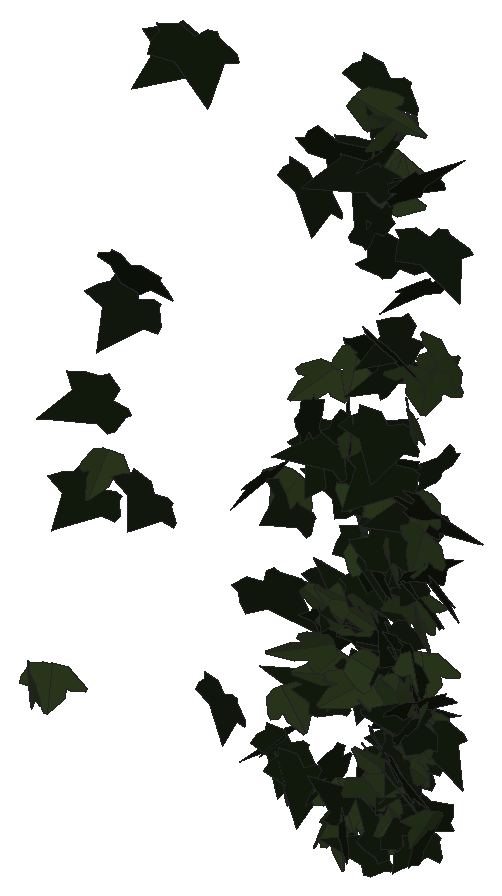
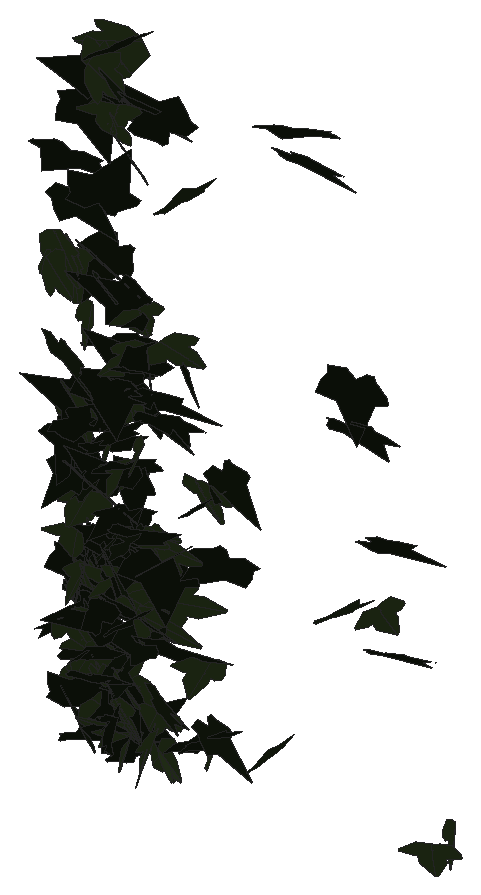
# SketchUp Ruby script. Lengths in inches.
U = 1.inch
M = Sketchup.active_model
def pt(a) = Geom::Point3d.new(a.map { |v| v * U })
def face(e, loops, mat)
  f = e.add_face(loops[0].map { |a| pt(a) })
  loops[1..].each { |l| e.add_face(l.map { |a| pt(a) }).erase! }
  f.material = f.back_material = mat if mat
  f
end
# faces: each face lists its corners as indices into pts; further lists are holes
def faces(e, pts, list, mat = nil) = list.each { |f| face(e, (f[0].is_a?(Array) ? f : [f]).map { |l| l.map { |i| pts[i] } }, mat) }
# xy, xz, yz: faces in a plane at the given z, y or x. An outline is a flat list of corners, or four numbers for a rectangle; further outlines are holes
def ring(l) = l.size == 4 ? [[l[0], l[1]], [l[2], l[1]], [l[2], l[3]], [l[0], l[3]]] : l.each_slice(2).to_a
def flat(e, list, mat, &to3) = list.each { |f| face(e, (f[0].is_a?(Array) ? f : [f]).map { |l| ring(l).map { |u, v| to3.(u, v) } }, mat) }
def xy(e, z, list, mat = nil) = flat(e, list, mat) { |x, y| [x, y, z] }
def xz(e, y, list, mat = nil) = flat(e, list, mat) { |x, z| [x, y, z] }
def yz(e, x, list, mat = nil) = flat(e, list, mat) { |y, z| [x, y, z] }
def lines(e, pts, list) = list.each { |a, b| e.add_line(pt(pts[a]), pt(pts[b])) }
# prism: a flat outline (further loops are holes) pulled along v
def prism(e, loops, v, mat = nil)
  f = face(e, loops, mat); d = Geom::Vector3d.new(v.map { |x| x * U })
  f.pushpull(f.normal.samedirection?(d) ? d.length : -d.length)
end
def box(e, o, s, mat = nil) = prism(e, [[o, [o[0] + s[0], o[1], o[2]], [o[0] + s[0], o[1] + s[1], o[2]], [o[0], o[1] + s[1], o[2]]]], [0, 0, s[2]], mat)
def at(x, y, z, deg = 0) = Geom::Transformation.translation(pt([x, y, z])) * Geom::Transformation.rotation(ORIGIN, Z_AXIS, deg.degrees)
def axes(o, x, y, z) = Geom::Transformation.new([*x, 0, *y, 0, *z, 0, *pt(o).to_a, 1])
def part(name) = M.definitions.add(name)
# library, detail: a bought-in or finely detailed component or shape, given as its bounding box
def library(name, o, s) = part(name).tap { |d| box(d.entities, o, s) }
def detail(e, o, s) = box(e.add_group.entities, o, s)
def put(e, d, t, mat = nil) = e.add_instance(d, t).tap { |i| i.material = mat if mat }
def group(e, t, mat = nil) = e.add_group.tap { |g| g.transformation = t; g.material = mat if mat }.entities
root = M.entities
M.materials.add("1026 AP 7946 SUNNY SIDE UP").color = [254, 231, 186]
M.materials.add("efeu1").color = [18, 25, 13]
M.materials.add("efeu2").color = [43, 57, 29]
c1 = part("ivyleaf_10")
p = [[0,0.5,-0.03],[-0.0625,2.02,-0.43],[-0.19,2.01,-0.46],[-0.54,1.05,-0.29],[-0.52,0.625,-0.18],[-0.83,0.76,-0.28],
  [-1.16,0.64,-0.33],[-1.15,0.33,-0.24],[-0.77,-0.39,0.02],[-0.3,-0.51,0.16],[0.04,-0.48,0.23],[-0.02,2.01,-0.4375],
  [-0.06,2.01,-0.43],[0.04,-0.49,0.23],[0.67,-0.49,0.14],[1.38,0.36,-0.2],[1.375,0.51,-0.24],[0.81,0.65,-0.19],
  [0.62,0.59,-0.15],[0.6,1.09,-0.28],[0.5,1.23,-0.31]]
faces(c1.entities,p,[[0,1,2,3,4,5,6,7,8,9,10],[11,12,0,13,14,15,16,17,18,19,20]],"efeu2")
c2 = part("ivyleaf_9")
p = [[1.54,2.16,1.25],[1.36,2.04,1.19],[-0.21,0.99,0.68],[-0.71,1.11,0.82],[-0.85,0.86,0.67],[-0.8,0.17,0.21],
  [-0.9,-0.01,0.1],[-0.67,-0.16,-0.02],[-0.08,-0.08,-0.05],[-0.03,-0.6,-0.4],[0.65,-0.88,-0.66],[0.83,-0.6,-0.49],
  [1.29,-0.42,-0.43],[1.8125,-0.07,-0.26],[1.21,0.44,0.15]]
faces(c2.entities,p,[[0,1,2,3,4,5,6,7,8,9,10,11,12,13,14]],"efeu1")
put(root,c1,axes([92.33,212.37,268.49],[-0.2245,0.20089,0.07802],[-0.1217,0.03523,-0.25018],[-0.3142,-0.15719,0.04116]),"1026 AP 7946 SUNNY SIDE UP")
put(root,c1,axes([92.34,212.78,268.375],[0.33952,0.1346,-0.0146],[-0.00256,-0.02554,-0.2614],[-0.21293,0.21493,-0.02015]),"1026 AP 7946 SUNNY SIDE UP")
put(root,c2,axes([93.01,212.95,271.36],[-0.37229,-0.12542,0.02519],[0.03074,-0.08778,-0.26181],[0.19877,-0.22133,0.08766]),"1026 AP 7946 SUNNY SIDE UP")
put(root,c2,axes([93.36,212.77,272.94],[-0.39245,-0.03965,0.11469],[-0.15828,-0.06595,-0.25654],[0.09799,-0.26531,0.04495]),"1026 AP 7946 SUNNY SIDE UP")
put(root,c1,axes([93.23,212.85,271.94],[0.17666,0.21288,-0.13628],[-0.10985,-0.114,-0.24852],[-0.37953,0.13209,0.0085]),"1026 AP 7946 SUNNY SIDE UP")
put(root,c2,axes([93.82,212.76,274.65],[-0.41495,-0.09449,-0.05067],[0.08225,-0.0021,-0.28809],[0.14548,-0.26834,0.01833]),"1026 AP 7946 SUNNY SIDE UP")
put(root,c2,axes([93.89,212.59,275.27],[0.3169,0.08749,-0.19105],[-0.28227,-0.05181,-0.22586],[-0.15727,0.26927,0.02042]),"1026 AP 7946 SUNNY SIDE UP")
put(root,c2,axes([93.97,212.9375,271.63],[-0.19027,-0.1939,0.14979],[0.00656,-0.16529,-0.22279],[0.38208,-0.09372,0.07842]),"1026 AP 7946 SUNNY SIDE UP")
put(root,c2,axes([94.69,212.91,278.76],[-0.47032,-0.03817,-0.00117],[0.0129,-0.05717,-0.30522],[0.05864,-0.2936,0.05778]),"1026 AP 7946 SUNNY SIDE UP")
put(root,c2,axes([94.875,212.71,279.06],[-0.18963,-0.26352,-0.0937],[0.21641,0.02826,-0.27674],[0.38032,-0.14747,0.11075]),"1026 AP 7946 SUNNY SIDE UP")
put(root,c2,axes([95.16,212.97,268.9375],[-0.02039,-0.23107,0.12399],[0.00467,-0.12194,-0.23897],[0.4106,-0.01009,0.00888]),"1026 AP 7946 SUNNY SIDE UP")
put(root,c2,axes([96.26,212.56,272.94],[-0.13618,0.20476,-0.14652],[0.07114,-0.13333,-0.23714],[-0.41456,-0.09014,0.00744]),"1026 AP 7946 SUNNY SIDE UP")
put(root,c2,axes([96.4,212.71,268.86],[-0.20709,0.20894,-0.0856],[0.01641,-0.09186,-0.25195],[-0.35387,-0.12653,0.03841]),"1026 AP 7946 SUNNY SIDE UP")
put(root,c1,axes([96.47,212.8125,272.77],[0.39388,-0.09084,-0.05273],[-0.08745,-0.00009,-0.26603],[0.15096,0.23696,-0.01652]),"1026 AP 7946 SUNNY SIDE UP")
put(root,c2,axes([96.42,212.82,268.7],[-0.13519,-0.24131,0.04194],[-0.00921,-0.04256,-0.264],[0.38505,-0.08574,0.00841]),"1026 AP 7946 SUNNY SIDE UP")
put(root,c1,axes([96.45,212.57,268.54],[-0.14579,0.23334,-0.05181],[0.0058,-0.05345,-0.26646],[-0.40558,-0.08464,0.01481]),"1026 AP 7946 SUNNY SIDE UP")
put(root,c2,axes([96.5625,212.86,272.41],[-0.18835,-0.12114,0.19483],[-0.12252,-0.17416,-0.17218],[0.35267,-0.1252,0.04424]),"1026 AP 7946 SUNNY SIDE UP")
put(root,c2,axes([96.41,212.3125,271.4],[-0.04255,-0.09695,-0.255],[0.13273,0.22379,-0.10376],[0.4138,-0.08175,0.00706]),"1026 AP 7946 SUNNY SIDE UP")
put(root,c1,axes([96.65,212.47,269.68],[0.20372,0.21474,0.10415],[0.03192,0.09698,-0.26019],[-0.39698,0.118,0.03252]),"1026 AP 7946 SUNNY SIDE UP")
put(root,c2,axes([96.71,212.98,277.36],[-0.0734,-0.25993,0.14131],[0.04415,-0.14366,-0.26857],[0.46111,-0.02762,0.04821]),"1026 AP 7946 SUNNY SIDE UP")
put(root,c2,axes([96.79,212.66,268.51],[-0.12131,-0.25965,0.0267],[-0.00107,-0.02836,-0.27911],[0.41055,-0.0768,0.00716]),"1026 AP 7946 SUNNY SIDE UP")
put(root,c1,axes([97.17,212.56,270.58],[0.02809,0.07874,-0.27569],[-0.36319,-0.14695,-0.06119],[-0.24714,0.2249,0.05858]),"1026 AP 7946 SUNNY SIDE UP")
put(root,c2,axes([97.37,212.73,269.83],[-0.23699,0.10731,0.21715],[-0.36103,-0.00907,-0.1649],[-0.08572,-0.25847,0.09416]),"1026 AP 7946 SUNNY SIDE UP")
put(root,c2,axes([97.15,212.31,274.0625],[0.08188,0.00079,0.30189],[-0.02346,0.28573,0.00566],[-0.47809,-0.01389,0.05143]),"1026 AP 7946 SUNNY SIDE UP")
put(root,c1,axes([97.19,212.67,274.74],[0.22421,0.11954,-0.19783],[-0.24235,-0.11986,-0.19232],[-0.28724,0.19443,0.00784]),"1026 AP 7946 SUNNY SIDE UP")
put(root,c1,axes([97.52,212.6875,270.1875],[-0.12567,0.04787,0.27433],[-0.3968,-0.11261,-0.05789],[0.15228,-0.25392,0.07556]),"1026 AP 7946 SUNNY SIDE UP")
put(root,c1,axes([97.5,212.43,271.27],[0.13878,0.01636,0.27818],[-0.43878,0.0358,0.08522],[-0.0498,-0.26983,0.02433]),"1026 AP 7946 SUNNY SIDE UP")
put(root,c2,axes([97.17,212.95,271.33],[-0.12762,-0.22357,0.13544],[-0.0188,-0.1357,-0.24378],[0.4084,-0.07611,0.0311]),"1026 AP 7946 SUNNY SIDE UP")
put(root,c2,axes([97.3,212.75,273.57],[-0.37125,-0.1217,-0.034],[0.06358,-0.00552,-0.2669],[0.20312,-0.2207,0.0214]),"1026 AP 7946 SUNNY SIDE UP")
put(root,c1,axes([97.29,212.62,268.07],[0.13289,-0.21436,0.11813],[0.04504,-0.11307,-0.23765],[0.38051,0.08825,-0.01313]),"1026 AP 7946 SUNNY SIDE UP")
put(root,c2,axes([97.61,212.62,273.73],[-0.38251,-0.00321,0.1396],[-0.21905,-0.03311,-0.23997],[0.03284,-0.25825,0.02536]),"1026 AP 7946 SUNNY SIDE UP")
put(root,c2,axes([97.41,212.55,271.09],[0.27984,0.16014,-0.15327],[-0.16085,-0.10985,-0.24701],[-0.30484,0.20497,-0.01037]),"1026 AP 7946 SUNNY SIDE UP")
put(root,c2,axes([97.4375,212.64,268.93],[-0.30467,0.04867,-0.17549],[0.21529,-0.11968,-0.19605],[-0.17745,-0.22876,0.06346]),"1026 AP 7946 SUNNY SIDE UP")
put(root,c1,axes([97.58,212.67,270.22],[-0.04372,-0.23313,0.13138],[-0.01523,-0.12858,-0.24257],[0.41856,-0.02903,0.0049]),"1026 AP 7946 SUNNY SIDE UP")
put(root,c1,axes([97.55,212.6,268.25],[-0.07758,0.24147,0.06883],[-0.0443,0.05718,-0.26184],[-0.42052,-0.05057,0.01489]),"1026 AP 7946 SUNNY SIDE UP")
put(root,c2,axes([97.91,212.33,273.38],[-0.14455,-0.01724,-0.27347],[-0.43422,0.00431,0.09112],[-0.0023,0.26901,-0.01521]),"1026 AP 7946 SUNNY SIDE UP")
put(root,c2,axes([97.3,212.57,278.15],[-0.01598,-0.03211,0.28796],[0.40968,-0.12415,-0.00855],[0.21042,0.23927,0.0385]),"1026 AP 7946 SUNNY SIDE UP")
put(root,c1,axes([97.98,212.4375,271.34],[-0.13113,-0.00069,-0.26805],[-0.40744,0.07477,0.0801],[0.12095,0.25112,-0.02078]),"1026 AP 7946 SUNNY SIDE UP")
put(root,c1,axes([97.46,212.5,267.92],[0.25294,-0.08245,0.19553],[0.24765,-0.10807,-0.18605],[0.2121,0.2245,-0.01596]),"1026 AP 7946 SUNNY SIDE UP")
put(root,c2,axes([97.9375,212.6,271.37],[-0.36797,-0.10691,-0.06061],[-0.10116,-0.00345,0.25757],[-0.17746,0.22366,-0.02116]),"1026 AP 7946 SUNNY SIDE UP")
put(root,c1,axes([97.66,212.73,275.14],[0.22568,0.19902,-0.09446],[-0.05589,-0.08687,-0.25659],[-0.36713,0.13556,-0.01901]),"1026 AP 7946 SUNNY SIDE UP")
put(root,c2,axes([97.875,212.55,268.25],[0.07744,0.03598,0.26717],[-0.40962,-0.06566,0.05655],[0.12136,-0.24457,0.02038]),"1026 AP 7946 SUNNY SIDE UP")
put(root,c2,axes([97.8,212.35,273.97],[0.00073,-0.01341,0.29449],[0.0458,0.27393,0.01807],[-0.46555,0.02693,0.00224]),"1026 AP 7946 SUNNY SIDE UP")
put(root,c1,axes([97.56,212.47,268.57],[0.35744,0.10985,0.07714],[0.11206,0.02306,-0.25976],[-0.17582,0.23803,-0.00873]),"1026 AP 7946 SUNNY SIDE UP")
put(root,c2,axes([97.74,212.33,268.16],[0.16499,-0.10004,-0.23734],[-0.28613,0.14094,-0.14797],[0.27104,0.20968,-0.01172]),"1026 AP 7946 SUNNY SIDE UP")
put(root,c2,axes([97.42,212.76,269.9375],[0.27998,-0.17999,0.12194],[0.14056,-0.07945,-0.26119],[0.30917,0.19911,0.00831]),"1026 AP 7946 SUNNY SIDE UP")
put(root,c1,axes([97.91,212.48,270.3],[0.29811,0.07186,-0.19269],[-0.27079,-0.08655,-0.20377],[-0.18941,0.23682,-0.01195]),"1026 AP 7946 SUNNY SIDE UP")
put(root,c2,axes([97.73,212.94,270.2],[-0.11311,-0.24046,0.09775],[-0.02563,-0.09549,-0.25888],[0.40646,-0.07294,0.01088]),"1026 AP 7946 SUNNY SIDE UP")
put(root,c1,axes([97.76,212.625,272.83],[-0.13712,0.22891,-0.05193],[0.0234,-0.04974,-0.26055],[-0.39761,-0.08187,0.00258]),"1026 AP 7946 SUNNY SIDE UP")
put(root,c2,axes([98.13,212.77,270.3],[-0.34632,0.09057,0.09423],[-0.15669,0.00395,-0.23651],[-0.14428,-0.22169,0.03067]),"1026 AP 7946 SUNNY SIDE UP")
put(root,c2,axes([98.01,212.65,268.95],[0.18066,-0.01885,-0.24291],[-0.38592,-0.00186,-0.11414],[0.01074,0.25038,-0.01562]),"1026 AP 7946 SUNNY SIDE UP")
put(root,c2,axes([98.18,212.57,278.32],[-0.48078,0.01511,0.07601],[-0.1223,-0.0305,-0.30197],[-0.01217,-0.29034,0.03157]),"1026 AP 7946 SUNNY SIDE UP")
put(root,c1,axes([98.08,212.67,268.57],[0.13697,-0.07937,-0.21137],[-0.21651,0.1496,-0.11873],[0.2871,0.15068,0.0113]),"1026 AP 7946 SUNNY SIDE UP")
put(root,c1,axes([97.97,212.61,268.14],[-0.2001,0.19179,0.09097],[-0.08478,0.06605,-0.23995],[-0.3441,-0.1278,0.00622]),"1026 AP 7946 SUNNY SIDE UP")
put(root,c1,axes([98.21,212.59,268.92],[0.01694,0.0539,0.24464],[-0.3655,0.09163,-0.01184],[-0.15601,-0.20881,0.05429]),"1026 AP 7946 SUNNY SIDE UP")
put(root,c2,axes([98.2,212.4,277.43],[-0.01796,0.14333,0.27703],[-0.12752,0.24723,-0.14753],[-0.48282,-0.07062,0.02866]),"1026 AP 7946 SUNNY SIDE UP")
put(root,c2,axes([98.05,212.4,272.27],[0.29062,-0.01238,-0.20738],[-0.32923,-0.01025,-0.1831],[0.00086,0.2582,-0.0136]),"1026 AP 7946 SUNNY SIDE UP")
put(root,c2,axes([98.25,212.61,268.72],[-0.15061,0.00594,-0.24946],[-0.37331,0.08077,0.09294],[0.13157,0.23597,-0.02185]),"1026 AP 7946 SUNNY SIDE UP")
put(root,c2,axes([98.23,212.56,267.75],[-0.15275,0.00133,0.22501],[-0.31495,-0.1079,-0.08582],[0.1676,-0.20155,0.04381]),"1026 AP 7946 SUNNY SIDE UP")
put(root,c2,axes([97.84,212.75,271.37],[0.13454,-0.21058,0.09113],[0.04691,-0.08348,-0.24202],[0.3845,0.08387,-0.00236]),"1026 AP 7946 SUNNY SIDE UP")
put(root,c2,axes([97.99,212.98,279.41],[-0.15713,-0.27607,0.09189],[-0.00465,-0.09501,-0.30162],[0.45693,-0.0959,0.02853]),"1026 AP 7946 SUNNY SIDE UP")
put(root,c2,axes([98.1875,212.53,270.59],[0.03281,0.09855,0.25777],[-0.03931,0.23985,-0.10032],[-0.43786,-0.01415,0.02832]),"1026 AP 7946 SUNNY SIDE UP")
put(root,c2,axes([98.24,212.73,272.89],[-0.17601,-0.22332,0.00079],[0.00382,0.00298,0.26364],[-0.37913,0.10371,0.00229]),"1026 AP 7946 SUNNY SIDE UP")
put(root,c2,axes([97.9,212.7,271.82],[-0.00015,-0.16732,-0.19499],[0.06041,0.17805,-0.17477],[0.41272,-0.02612,0.02551]),"1026 AP 7946 SUNNY SIDE UP")
put(root,c2,axes([97.72,212.73,275.22],[0.29054,0.0367,-0.19928],[0.26229,0.11957,0.17855],[0.18827,-0.22321,0.05879]),"1026 AP 7946 SUNNY SIDE UP")
put(root,c2,axes([98.0625,212.47,271.12],[0.3483,0.10535,-0.10958],[-0.13214,-0.07388,-0.24619],[-0.21338,0.21771,-0.02641]),"1026 AP 7946 SUNNY SIDE UP")
put(root,c2,axes([97.85,212.43,274],[-0.0821,-0.00054,0.27652],[0.43847,-0.00049,0.05177],[0.00065,0.26279,0.00433]),"1026 AP 7946 SUNNY SIDE UP")
put(root,c2,axes([97.99,212.6,272.5],[-0.12105,-0.22727,-0.0918],[0.06234,0.07513,-0.25364],[0.40583,-0.07933,0.01158]),"1026 AP 7946 SUNNY SIDE UP")
put(root,c1,axes([98.06,212.35,273.17],[0.23019,0.20757,-0.09751],[0.06924,0.08525,0.26633],[0.3804,-0.14112,0.01053]),"1026 AP 7946 SUNNY SIDE UP")
put(root,c1,axes([98.31,212.62,269],[-0.23164,-0.07138,-0.18921],[-0.26803,-0.07737,0.16375],[-0.17862,0.20867,-0.00036]),"1026 AP 7946 SUNNY SIDE UP")
put(root,c1,axes([97.95,212.38,274.22],[-0.16194,-0.13614,-0.22458],[0.27061,0.13745,-0.17267],[0.32381,-0.18295,0.03199]),"1026 AP 7946 SUNNY SIDE UP")
put(root,c1,axes([97.98,212.46,272.39],[0.16529,0.21811,0.12436],[0.09841,0.09807,-0.25404],[-0.40547,0.11271,-0.01096]),"1026 AP 7946 SUNNY SIDE UP")
put(root,c1,axes([98.04,212.77,278.29],[0.34514,0.1697,0.02597],[0.05541,-0.00486,-0.28237],[-0.28515,0.20445,-0.02344]),"1026 AP 7946 SUNNY SIDE UP")
put(root,c2,axes([98.33,212.625,278.76],[-0.31602,0.1593,-0.1062],[0.11384,-0.07715,-0.26297],[-0.29954,-0.19739,0.0121]),"1026 AP 7946 SUNNY SIDE UP")
put(root,c1,axes([97.94,212.51,270.59],[0.15317,0.12675,0.22455],[0.22285,0.16165,-0.16409],[-0.34845,0.1591,-0.00624]),"1026 AP 7946 SUNNY SIDE UP")
put(root,c2,axes([98.25,212.64,273.75],[0.20479,0.19583,-0.10198],[-0.09646,-0.07983,-0.24727],[-0.35885,0.13322,0.00827]),"1026 AP 7946 SUNNY SIDE UP")
put(root,c1,axes([98.28,212.9,278.875],[-0.0139,-0.24347,0.18886],[-0.01402,-0.1845,-0.25206],[0.48033,-0.01243,-0.00189]),"1026 AP 7946 SUNNY SIDE UP")
put(root,c2,axes([98.32,212.79,276.74],[0.23643,0.06825,0.24488],[-0.37945,-0.05268,0.16244],[0.13798,-0.2618,0.0271]),"1026 AP 7946 SUNNY SIDE UP")
put(root,c2,axes([97.99,212.625,269.16],[0.30994,-0.17209,0.04239],[0.02965,-0.0423,-0.26846],[0.29917,0.18247,-0.01731]),"1026 AP 7946 SUNNY SIDE UP")
put(root,c2,axes([98.37,212.66,268.05],[0.04648,-0.07934,0.24521],[-0.03855,0.22968,0.0909],[-0.41133,-0.03049,0.01919]),"1026 AP 7946 SUNNY SIDE UP")
put(root,c1,axes([98.15,212.4,268.89],[-0.35619,-0.09086,-0.13856],[0.2077,0.02948,-0.25049],[0.14716,-0.26153,0.01817]),"1026 AP 7946 SUNNY SIDE UP")
put(root,c2,axes([98.48,212.51,275.28],[-0.32418,0.16834,-0.03663],[0.0221,-0.04009,-0.27215],[-0.29153,-0.19023,0.02009]),"1026 AP 7946 SUNNY SIDE UP")
put(root,c1,axes([98.375,212.68,278.86],[-0.2048,-0.15129,-0.21932],[-0.15663,-0.183,0.20228],[-0.40006,0.1491,0.03308]),"1026 AP 7946 SUNNY SIDE UP")
put(root,c2,axes([98.41,212.55,273.8],[-0.37018,-0.16855,0.05862],[-0.05739,-0.04823,-0.29801],[0.27426,-0.23758,0.01676]),"1026 AP 7946 SUNNY SIDE UP")
put(root,c2,axes([98.11,212.73,269.26],[0.04341,-0.13844,0.18917],[0.06102,-0.17486,-0.15313],[0.37858,0.04406,0.00299]),"1026 AP 7946 SUNNY SIDE UP")
put(root,c2,axes([98.43,212.38,268.04],[-0.15538,-0.19336,0.10242],[0.05357,0.09357,0.23006],[-0.36422,0.09625,-0.00986]),"1026 AP 7946 SUNNY SIDE UP")
put(root,c1,axes([98.04,212.56,268.1],[0.20119,-0.03567,-0.23927],[0.3512,0.09994,0.11163],[0.11377,-0.24542,0.07853]),"1026 AP 7946 SUNNY SIDE UP")
put(root,c1,axes([98.23,212.65,277.84],[0.46752,-0.07897,-0.0181],[0.044,0.03334,0.30432],[-0.12947,-0.27384,0.03807]),"1026 AP 7946 SUNNY SIDE UP")
put(root,c2,axes([98.375,212.9,269.1],[-0.34021,-0.15496,-0.02032],[0.08352,-0.0428,-0.26597],[0.23082,-0.21292,0.06629]),"1026 AP 7946 SUNNY SIDE UP")
put(root,c1,axes([98.04,212.51,279.27],[-0.19659,-0.02439,-0.27308],[0.4344,-0.01497,-0.12321],[-0.0061,-0.27944,0.0265]),"1026 AP 7946 SUNNY SIDE UP")
put(root,c2,axes([98.56,212.69,275.76],[-0.41814,0.09069,-0.04531],[0.05255,-0.04113,-0.28004],[-0.16246,-0.24673,0.02602]),"1026 AP 7946 SUNNY SIDE UP")
put(root,c2,axes([98.34,212.51,274.39],[-0.25368,-0.2092,-0.01923],[0.03853,0.00247,-0.2746],[0.35398,-0.15019,0.01611]),"1026 AP 7946 SUNNY SIDE UP")
put(root,c2,axes([98.1875,212.5625,272.11],[-0.14638,0.02239,0.25917],[0.41198,0.0165,0.09126],[-0.01373,0.25618,-0.02491]),"1026 AP 7946 SUNNY SIDE UP")
put(root,c2,axes([98.6875,212.37,268.32],[-0.1218,0.16726,0.18353],[-0.18834,0.13286,-0.18907],[-0.35733,-0.12704,0.0371]),"1026 AP 7946 SUNNY SIDE UP")
put(root,c1,axes([98.48,212.66,268.54],[0.16808,0.1525,-0.17423],[-0.15592,-0.13676,-0.19656],[-0.34772,0.13505,0.00392]),"1026 AP 7946 SUNNY SIDE UP")
put(root,c2,axes([98.34,212.625,271.07],[-0.03661,-0.14612,0.25254],[-0.04038,-0.24472,-0.1537],[0.44804,-0.03399,0.00678]),"1026 AP 7946 SUNNY SIDE UP")
put(root,c2,axes([98.54,212.36,272.49],[-0.31765,-0.10791,0.13956],[0.16939,0.08917,0.23114],[-0.2343,0.21077,-0.0221]),"1026 AP 7946 SUNNY SIDE UP")
put(root,c2,axes([98.31,212.63,271.22],[-0.2243,-0.09929,-0.20531],[0.29255,0.08449,-0.17395],[0.21765,-0.21587,0.02224]),"1026 AP 7946 SUNNY SIDE UP")
put(root,c2,axes([98.39,212.35,275.75],[0.41826,-0.01382,-0.14852],[-0.22072,0.04893,-0.27151],[0.05554,0.29853,0.03942]),"1026 AP 7946 SUNNY SIDE UP")
put(root,c2,axes([98.61,212.6875,278.18],[0.07489,0.23288,-0.11607],[-0.04714,-0.10813,-0.25517],[-0.43573,0.05172,0.00766]),"1026 AP 7946 SUNNY SIDE UP")
put(root,c2,axes([98.54,212.86,269.42],[-0.29893,-0.18855,0.00457],[0.01286,-0.01605,-0.27537],[0.29633,-0.18951,0.01656]),"1026 AP 7946 SUNNY SIDE UP")
put(root,c2,axes([98.24,212.88,270.06],[0.05663,-0.11505,0.24777],[0.20345,-0.2054,-0.12206],[0.3676,0.13141,0.02938]),"1026 AP 7946 SUNNY SIDE UP")
put(root,c2,axes([98.8125,212.66,272.13],[-0.31371,0.18002,0.07465],[-0.12433,0.01792,-0.2739],[-0.27801,-0.21115,0.03826]),"1026 AP 7946 SUNNY SIDE UP")
put(root,c1,axes([98.54,212.31,272.59],[-0.17221,0.22235,0.07196],[-0.06121,0.05419,-0.26068],[-0.38813,-0.1072,0.00918]),"1026 AP 7946 SUNNY SIDE UP")
put(root,c2,axes([98.37,212.6,269.96],[0.04131,0.1172,-0.2309],[0.04475,0.21578,0.13082],[0.41657,-0.0348,0.00884]),"1026 AP 7946 SUNNY SIDE UP")
put(root,c1,axes([98.82,212.35,270.56],[-0.127,0.11656,0.21117],[-0.30654,0.09524,-0.13329],[-0.23575,-0.18664,0.05956]),"1026 AP 7946 SUNNY SIDE UP")
put(root,c1,axes([98.55,212.66,269.39],[-0.3486,-0.10154,-0.08743],[0.14373,0.00865,-0.24328],[0.16629,-0.22034,0.02701]),"1026 AP 7946 SUNNY SIDE UP")
put(root,c2,axes([98.78,212.86,273.09],[-0.01352,-0.09609,-0.26073],[-0.05329,-0.24028,0.09977],[-0.43924,0.03211,-0.00408]),"1026 AP 7946 SUNNY SIDE UP")
put(root,c2,axes([98.49,212.73,269.42],[0.01101,-0.23338,-0.00754],[-0.00266,0.00396,-0.24989],[0.39622,0.00651,-0.00147]),"1026 AP 7946 SUNNY SIDE UP")
put(root,c2,axes([98.65,212.86,268.09],[-0.21592,-0.17245,0.06598],[-0.04678,-0.05892,-0.22986],[0.30866,-0.12957,0.01132]),"1026 AP 7946 SUNNY SIDE UP")
put(root,c2,axes([98.76,212.7,268.43],[0.25353,0.00694,0.21434],[-0.3201,0.08885,0.14861],[-0.11435,-0.23336,0.05922]),"1026 AP 7946 SUNNY SIDE UP")
put(root,c1,axes([98.41,212.54,270.41],[-0.23244,0.00811,-0.22407],[0.33054,-0.08753,-0.14117],[-0.13148,-0.23439,0.04123]),"1026 AP 7946 SUNNY SIDE UP")
put(root,c1,axes([98.74,212.54,274.7],[-0.25572,0.18715,0.08434],[-0.11127,0.04483,-0.25551],[-0.32457,-0.16282,0.02114]),"1026 AP 7946 SUNNY SIDE UP")
put(root,c2,axes([98.87,212.41,271.01],[0.11753,-0.0255,-0.25852],[-0.41149,-0.00055,-0.07445],[0.01104,0.25089,-0.0229]),"1026 AP 7946 SUNNY SIDE UP")
put(root,c2,axes([99.03,212.4,270.11],[-0.12347,-0.0481,-0.25694],[-0.38489,-0.07935,0.08972],[-0.15375,0.23726,-0.01826]),"1026 AP 7946 SUNNY SIDE UP")
put(root,c1,axes([98.76,212.88,269.88],[-0.24732,-0.18303,0.12366],[0.00387,-0.15043,-0.23184],[0.34504,-0.1295,0.09124]),"1026 AP 7946 SUNNY SIDE UP")
put(root,c2,axes([98.88,212.74,276.69],[-0.10634,0.1813,-0.17593],[-0.01576,-0.17361,-0.20084],[-0.41778,-0.0396,0.05236]),"1026 AP 7946 SUNNY SIDE UP")
put(root,c2,axes([98.45,212.52,269.125],[0.13807,-0.12964,0.20706],[0.13896,-0.17778,-0.16548],[0.37257,0.11435,-0.01501]),"1026 AP 7946 SUNNY SIDE UP")
put(root,c1,axes([98.6875,212.63,271.77],[-0.34379,-0.1076,-0.08627],[0.13127,0.02283,-0.24466],[0.18492,-0.21625,0.0133]),"1026 AP 7946 SUNNY SIDE UP")
put(root,c2,axes([98.8125,212.5,270.7],[0.15696,-0.06304,-0.25907],[-0.32849,0.13937,-0.12078],[0.24048,0.23152,0.00412]),"1026 AP 7946 SUNNY SIDE UP")
put(root,c1,axes([98.59,212.66,269.21],[0.00527,-0.07276,-0.24727],[0.22086,-0.19322,0.06462],[-0.34488,-0.12485,0.0376]),"1026 AP 7946 SUNNY SIDE UP")
put(root,c2,axes([98.6875,212.62,267.9375],[-0.04207,0.19924,0.16422],[0.02239,-0.15028,0.2128],[0.42358,0.02774,0.00506]),"1026 AP 7946 SUNNY SIDE UP")
put(root,c2,axes([98.91,212.2,270.03],[0.05461,0.12058,0.22275],[0.0185,0.2074,-0.12858],[-0.4055,0.0257,0.02413]),"1026 AP 7946 SUNNY SIDE UP")
put(root,c2,axes([98.83,212.69,271.81],[0.25377,-0.21362,-0.03621],[0.05263,-0.01611,0.27838],[-0.36263,-0.15183,0.01506]),"1026 AP 7946 SUNNY SIDE UP")
put(root,c1,axes([98.9,212.5,270.42],[0.00796,0.16228,0.18858],[-0.09064,0.17035,-0.16614],[-0.39364,-0.03594,0.04207]),"1026 AP 7946 SUNNY SIDE UP")
put(root,c1,axes([98.96,212.4375,270.42],[0.2137,-0.20671,-0.07537],[-0.08025,0.05035,-0.25799],[0.36042,0.13378,-0.01276]),"1026 AP 7946 SUNNY SIDE UP")
put(root,c1,axes([98.9,212.66,273.34],[0.34847,-0.14698,-0.00027],[-0.01841,-0.01798,-0.26961],[0.24884,0.20449,-0.01956]),"1026 AP 7946 SUNNY SIDE UP")
put(root,c2,axes([98.78,212.25,278.3],[0.06574,0.24479,-0.13517],[-0.03759,0.13303,0.26408],[0.46856,-0.02367,0.04015]),"1026 AP 7946 SUNNY SIDE UP")
put(root,c1,axes([98.99,212.48,269.95],[0.30558,-0.16068,-0.05425],[-0.08015,0.01989,-0.25745],[0.27344,0.18539,-0.01483]),"1026 AP 7946 SUNNY SIDE UP")
put(root,c1,axes([99.0625,212.39,272.95],[-0.39427,0.11763,0.05354],[-0.13483,-0.06979,-0.2673],[-0.15013,-0.24624,0.09945]),"1026 AP 7946 SUNNY SIDE UP")
put(root,c1,axes([99.03,212.46,271.37],[-0.24697,0.18994,-0.03752],[-0.0202,0.03808,0.25627],[0.32805,0.14534,-0.01247]),"1026 AP 7946 SUNNY SIDE UP")
put(root,c1,axes([99.06,212.51,275.41],[-0.41532,-0.14244,0.0406],[-0.03583,-0.04216,-0.30823],[0.22996,-0.26383,0.0253]),"1026 AP 7946 SUNNY SIDE UP")
put(root,c2,axes([99.04,212.29,270.48],[0.11886,0.24678,-0.03771],[-0.01596,-0.03729,-0.27514],[-0.42367,0.07064,-0.00022]),"1026 AP 7946 SUNNY SIDE UP")
put(root,c2,axes([98.88,212.71,272.19],[0.35257,-0.07228,-0.10066],[-0.15436,0.02168,-0.23495],[0.12725,0.22656,-0.00611]),"1026 AP 7946 SUNNY SIDE UP")
put(root,c1,axes([99.22,212.65,275.7],[-0.33584,0.11381,0.17068],[-0.28507,-0.00675,-0.23697],[-0.13452,-0.26983,0.07605]),"1026 AP 7946 SUNNY SIDE UP")
put(root,c2,axes([99.2,212.58,274],[-0.15225,0.22314,0.07389],[-0.06179,0.05653,-0.25634],[-0.39021,-0.09602,0.01176]),"1026 AP 7946 SUNNY SIDE UP")
put(root,c1,axes([99.09,212.48,275.57],[0.20609,-0.21686,-0.06737],[-0.05671,0.05016,-0.26533],[0.37777,0.12583,-0.00308]),"1026 AP 7946 SUNNY SIDE UP")
put(root,c2,axes([98.86,212.82,269.83],[0.02878,-0.25581,-0.0871],[0.05788,0.08488,-0.26037],[0.41895,0.00585,0.04195]),"1026 AP 7946 SUNNY SIDE UP")
put(root,c1,axes([99.1,212.46,268.67],[-0.07516,-0.20635,0.09155],[-0.01643,-0.08807,-0.227],[0.3806,-0.04455,0.00828]),"1026 AP 7946 SUNNY SIDE UP")
put(root,c2,axes([99.03,212.4,272.49],[0.17537,0.22011,0.05802],[0.06406,0.03884,-0.25911],[-0.37829,0.10862,-0.01698]),"1026 AP 7946 SUNNY SIDE UP")
put(root,c1,axes([99.08,212.89,275.45],[-0.00689,-0.26548,0.12711],[0.02519,-0.12494,-0.27374],[0.46063,0.00286,0.01687]),"1026 AP 7946 SUNNY SIDE UP")
put(root,c2,axes([98.875,212.79,277.34],[-0.17438,-0.14942,-0.19703],[0.26106,0.10793,-0.18619],[0.30288,-0.17906,0.04704]),"1026 AP 7946 SUNNY SIDE UP")
put(root,c2,axes([98.6875,212.59,273.21],[0.21998,-0.08857,0.23786],[0.30996,-0.12861,-0.16982],[0.26507,0.2239,0.00119]),"1026 AP 7946 SUNNY SIDE UP")
put(root,c1,axes([98.98,212.47,271.02],[0.34156,0.13013,0.0244],[0.04766,-0.00469,-0.25578],[-0.21865,0.20226,-0.01764]),"1026 AP 7946 SUNNY SIDE UP")
